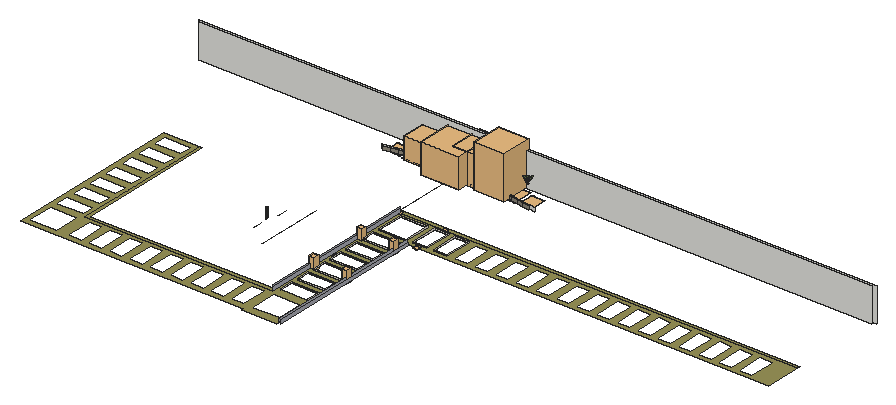
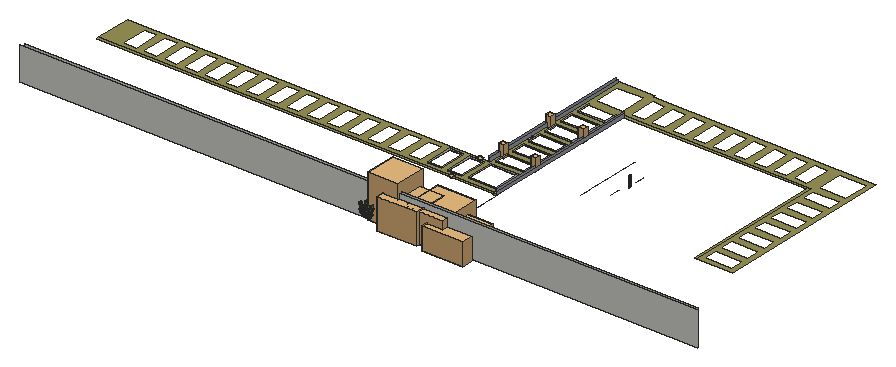
# SketchUp Ruby script. Lengths in inches.
U = 1.inch
M = Sketchup.active_model
def pt(a) = Geom::Point3d.new(a.map { |v| v * U })
def face(e, loops, mat)
  f = e.add_face(loops[0].map { |a| pt(a) })
  loops[1..].each { |l| e.add_face(l.map { |a| pt(a) }).erase! }
  f.material = f.back_material = mat if mat
  f
end
# faces: each face lists its corners as indices into pts; further lists are holes
def faces(e, pts, list, mat = nil) = list.each { |f| face(e, (f[0].is_a?(Array) ? f : [f]).map { |l| l.map { |i| pts[i] } }, mat) }
# xy, xz, yz: faces in a plane at the given z, y or x. An outline is a flat list of corners, or four numbers for a rectangle; further outlines are holes
def ring(l) = l.size == 4 ? [[l[0], l[1]], [l[2], l[1]], [l[2], l[3]], [l[0], l[3]]] : l.each_slice(2).to_a
def flat(e, list, mat, &to3) = list.each { |f| face(e, (f[0].is_a?(Array) ? f : [f]).map { |l| ring(l).map { |u, v| to3.(u, v) } }, mat) }
def xy(e, z, list, mat = nil) = flat(e, list, mat) { |x, y| [x, y, z] }
def xz(e, y, list, mat = nil) = flat(e, list, mat) { |x, z| [x, y, z] }
def yz(e, x, list, mat = nil) = flat(e, list, mat) { |y, z| [x, y, z] }
def lines(e, pts, list) = list.each { |a, b| e.add_line(pt(pts[a]), pt(pts[b])) }
# prism: a flat outline (further loops are holes) pulled along v
def prism(e, loops, v, mat = nil)
  f = face(e, loops, mat); d = Geom::Vector3d.new(v.map { |x| x * U })
  f.pushpull(f.normal.samedirection?(d) ? d.length : -d.length)
end
def box(e, o, s, mat = nil) = prism(e, [[o, [o[0] + s[0], o[1], o[2]], [o[0] + s[0], o[1] + s[1], o[2]], [o[0], o[1] + s[1], o[2]]]], [0, 0, s[2]], mat)
def at(x, y, z, deg = 0) = Geom::Transformation.translation(pt([x, y, z])) * Geom::Transformation.rotation(ORIGIN, Z_AXIS, deg.degrees)
def axes(o, x, y, z) = Geom::Transformation.new([*x, 0, *y, 0, *z, 0, *pt(o).to_a, 1])
def part(name) = M.definitions.add(name)
# library, detail: a bought-in or finely detailed component or shape, given as its bounding box
def library(name, o, s) = part(name).tap { |d| box(d.entities, o, s) }
def detail(e, o, s) = box(e.add_group.entities, o, s)
def put(e, d, t, mat = nil) = e.add_instance(d, t).tap { |i| i.material = mat if mat }
def group(e, t, mat = nil) = e.add_group.tap { |g| g.transformation = t; g.material = mat if mat }.entities
root = M.entities
M.materials.add("Marble_01_1K").color = [230, 221, 211]
M.materials.add("Marble_07_1K").color = [36, 34, 36]
M.materials.add("Marble_20_1K").color = [172, 173, 182]
M.materials.add("Material__4").color = [36, 36, 36]
M.materials.add("Material__6").color = [79, 108, 5]
M.materials.add("Plaster_06_1K").color = [141, 135, 122]
M.materials.add("Soil_04_1K").color = [152, 146, 88]
M.materials.add("calathea lutea").color = [121, 145, 80]
c1 = library("tt",[-12.4,-12.1,0],[24.8,24.2,0.01])
c2 = library("ew",[-14.92,-16.84,0],[29.84,33.68,0.01])
c3 = library("t1",[-17.79,-17.21,0],[35.58,34.42,0.01])
c4 = library("light",[-4,-4,0],[8,8,0.01])
c5 = library("Group\#54",[0,0,0],[2062.46,2062.46,4833.66])
c6 = part("Landscape+Light")
put(c6.entities,c5,at(-2096.57,-1031.23,-3775.98))
c7 = part("Group\#156")
g1 = group(c7.entities,at(8.61,38.85,0))
xy(g1,0,[[0,0,2.82,19.1,22.58,0],[22.58,0,2.82,19.1,22.58,19.1]],"calathea lutea")
p = [[2.82,19.1,0],[7.19,48.22,5.13],[10.77,48.22,5.13],[12.74,48.22,5.13],[22.58,48.22,5.13],[22.58,19.1,0]]
faces(g1,p,[[0,1,2,3,4,5]],"calathea lutea")
g2 = group(c7.entities,at(-0.77,-7.77,0))
p = [[14.8125,23.31,1.46],[21.35,23.31,0],[14.8125,0,1.46],[21.35,0,0],[27.89,0,1.46],[27.89,23.31,1.46],
  [8.27,46.62,2.92],[21.35,46.62,0],[34.4375,46.62,2.92],[4.47,23.31,6.43],[0,0,8.59],[33.76,0,4.28],
  [33.76,23.31,4.28]]
faces(g2,p,[[0,1,2],[3,2,1],[4,3,5],[1,5,3],[6,7,0],[1,0,7],[5,1,8],[7,8,1],
  [9,0,2,10],[11,4,5,12],[9,6,0],[12,5,8]],"calathea lutea")
c8 = part("Group\#150")
xy(c8.entities,0,[[0,0,0,33.87,27.21,33.87,19.71,0]],"calathea lutea")
c9 = part("Group\#157")
xy(c9.entities,1.04,[[21.13,33.87,21.13,57.59,32.375,57.59,27.12,33.87]],"calathea lutea")
xy(c9.entities,1.32,[[0.12,33.87,7.74,57.59]],"calathea lutea")
p = [[7.74,33.87,1.32],[11.8,57.59,0.61],[15.24,57.59,0],[15.24,33.87,0],[18.43,57.59,0.5625],[21.13,57.59,1.04],
  [21.13,33.87,1.04],[15.24,77.7,2.36],[21.13,77.7,3.4],[7.74,57.59,1.32],[7.74,77.7,3.69],[36.83,77.7,3.4],
  [32.375,57.59,1.04],[0.12,57.59,1.32],[0.12,77.7,3.69]]
faces(c9.entities,p,[[0,1,2,3],[3,2,4],[3,4,5,6],[7,2,1],[8,4,2,7],[0,9,1],[7,1,9,10],[8,5,4],
  [11,12,5,8],[10,9,13,14]],"calathea lutea")
put(c9.entities,c8,axes([0,-16.9375,0],[1,0,0],[0,1.5,0],[0,0,1]))
c10 = part("Group\#155")
g3 = group(c10.entities,at(0,-17.3,0))
xy(g3,0,[[0,0,28.07,51.9]],"calathea lutea")
g4 = group(c10.entities,at(0.9,34.6,0))
xy(g4,0,[[13.14,0,13.14,26.22,16.85,26.22],[13.14,0,16.85,26.22,20.16,26.22,20.16,0]],"calathea lutea")
p = [[6.36,0,1.82],[9.95,26.22,0.86],[13.14,26.22,0],[13.14,0,0],[20.16,0,0],[20.16,26.22,0],
  [27.07,26.22,1.22],[27.07,0,1.22],[13.14,49.5625,5.91],[20.16,49.5625,5.91],[16.85,26.22,0],[27.07,49.5625,7.125],
  [6.36,26.22,1.82],[6.36,49.5625,7.72],[0,0,4.78],[0,26.22,4.78],[0,49.5625,10.6875]]
faces(g4,p,[[0,1,2,3],[4,5,6,7],[8,2,1],[9,10,2,8],[9,5,10],[11,6,5,9],[0,12,1],[8,1,12,13],
  [14,15,12,0],[13,12,15,16]],"calathea lutea")
c11 = part("Group\#154")
put(c11.entities,c8,axes([0,-16.9375,0],[1,0,0],[0,1.5,0],[0,0,1]))
g5 = group(c11.entities,at(-0.23,33.4,-0.35))
p = [[15.12,39.14,-19.87],[15.12,20.54,-11.86],[11.68,20.84,-11.33],[21.02,39.66,-18.97],[18.3125,20.82,-11.37],[7.62,21.2,-10.71],
  [7.62,39.8,-18.72],[21.02,21.06,-10.96],[36.72,39.66,-18.97],[32.26,21.06,-10.96],[0,21.2,-10.71],[0,39.8,-18.72],
  [7.62,0.66,1.15],[15.12,0,0],[21.02,0.52,0.9],[27.01,0.52,0.9],[0,0.66,1.15]]
faces(g5,p,[[0,1,2],[3,4,1,0],[0,2,5,6],[3,7,4],[8,9,7,3],[6,5,10,11],[12,2,1,13],[13,1,4],
  [13,4,7,14],[12,5,2],[14,7,9,15],[16,10,5,12]],"calathea lutea")
c12 = part("Foliage cluster")
put(c12.entities,c7,axes([37.24,8.07,75.17],[1,0,0],[0,0.45554,-0.89021],[0,0.89021,0.45554]))
put(c12.entities,c9,axes([69.44,65.48,16.68],[-0.53288,-0.84619,0],[0.14694,-0.09253,0.98481],[-0.83334,0.52478,0.17365]))
put(c12.entities,c10,axes([47.9375,70.43,17.04],[0.74664,-0.66523,0],[0.11552,0.12965,0.98481],[-0.65512,-0.7353,0.17365]))
put(c12.entities,c7,axes([76.19,10.66,75.17],[0.70711,0.70711,0],[-0.32212,0.32212,-0.89021],[-0.62948,0.62948,0.45554]))
put(c12.entities,c7,axes([101.91,40.03,75.17],[0,1,0],[-0.45554,0,-0.89021],[-0.89021,0,0.45554]))
put(c12.entities,c7,axes([99.32,78.99,75.17],[-0.70711,0.70711,0],[-0.32212,-0.32212,-0.89021],[-0.62948,-0.62948,0.45554]))
put(c12.entities,c10,axes([34.81,63.36,17.04],[0.99956,-0.02967,0],[0.00515,0.17357,0.98481],[-0.02922,-0.98437,0.17365]))
put(c12.entities,c10,axes([48,37.4,15.8],[-0.14436,0.98953,0],[-0.40248,-0.05871,0.91355],[0.90398,0.13188,0.40674]))
put(c12.entities,c9,axes([56.87,39.77,12.28],[-0.67695,0.4263,0],[-0.18016,-0.28609,0.72505],[0.38636,0.61353,0.33809]))
put(c12.entities,c9,axes([36.12,43.25,12.28],[0.18947,0.77724,0],[-0.32848,0.08007,0.72505],[0.70442,-0.17172,0.33809]))
put(c12.entities,c11,axes([35.1,54.93,11.375],[0.79719,0.06694,0],[-0.03636,0.43302,0.6717],[0.05621,-0.66934,0.43454]))
put(c12.entities,c9,axes([41.66,47.32,12.28],[0.45082,0.66088,0],[-0.2793,0.19053,0.72505],[0.59896,-0.40858,0.33809]))
put(c12.entities,c9,axes([47.89,59.4,12.28],[0.79719,0.06694,0],[-0.02829,0.33691,0.72505],[0.06067,-0.7225,0.33809]))
put(c12.entities,c11,axes([29.53,49.96,11.375],[0.65692,0.45657,0],[-0.248,0.35682,0.6717],[0.38335,-0.55156,0.43454]))
put(c12.entities,c11,axes([29.9,49.27,12.86],[0.34062,0.72386,0],[-0.22849,0.10752,0.7591],[0.68685,-0.32321,0.25252]))
put(c12.entities,c11,axes([36.33,48.82,8.99],[0.09232,0.62522,0],[-0.3396,0.05015,0.53064],[0.52495,-0.07752,0.34329]))
put(c12.entities,c11,axes([49.82,38.52,8.99],[-0.54622,0.31791,0],[-0.17268,-0.29669,0.53064],[0.26692,0.45862,0.34329]))
put(c12.entities,c11,axes([55.68,39.21,8.99],[-0.632,0.00221,0],[-0.0012,-0.34328,0.53064],[0.00185,0.53064,0.34329]))
c13 = library("Group\#28",[0,0,0],[86.94,78.77,46.4375])
c14 = library("Group\#14",[-978.71,-103.24,719.12],[90.2,76.4,68.29])
c15 = library("Group\#13",[-906.16,-138.28,686.8],[98.25,106.18,75.79])
c16 = library("Group\#202",[-3.47,-2.45,12.47],[53.14,54.93,75.51])
xy(root,0,[[[498.69,562.78,561.69,562.78,561.69,850.66,1202.44,850.66,1202.44,913.66,498.69,913.66,498.69,632.1,166.21,632.1,166.21,885.25,103.21,885.25,103.21,567.28,498.69,567.28],[506.43,856.64,554.43,904.64],[506.43,576.78,554.43,624.64],[111.43,576.78,159.43,624.64],[506.43,820.64,554.43,844.64],[506.43,784.64,554.43,808.64],[506.43,748.64,554.43,772.64],[506.43,712.64,554.43,736.64],[506.43,676.64,554.43,700.64],[506.43,640.64,554.43,664.64],[468.08,576.64,492.08,624.64],[432.08,576.64,456.08,624.64],[396.08,576.64,420.08,624.64],[360.08,576.64,384.08,624.64],[324.08,576.64,348.08,624.64],[288.08,576.64,312.08,624.64],[252.08,576.64,276.08,624.64],[216.08,576.64,240.08,624.64],[180.08,576.64,204.08,624.64],[111.43,636.64,159.43,660.64],[111.43,672.64,159.43,696.64],[111.43,708.64,159.43,732.64],[111.43,744.64,159.43,768.64],[111.43,780.64,159.43,804.64],[111.43,816.64,159.43,840.64],[111.43,852.64,159.43,876.64],[1142.43,858.14,1166.43,906.14],[1106.43,858.14,1130.43,906.14],[1070.43,858.14,1094.43,906.14],[1034.43,858.14,1058.43,906.14],[998.43,858.14,1022.43,906.14],[962.43,858.14,986.43,906.14],[926.43,858.14,950.43,906.14],[890.43,858.14,914.43,906.14],[854.43,858.14,878.43,906.14],[818.43,858.14,842.43,906.14],[782.43,858.14,806.43,906.14],[746.43,858.14,770.43,906.14],[710.43,858.14,734.43,906.14],[674.43,858.14,698.43,906.14],[638.43,858.14,662.43,906.14],[602.43,858.14,626.43,906.14],[566.43,858.14,590.43,906.14]],[166.21,632.1,166.21,885.25,170.71,885.25,170.71,636.6,494.19,636.6,494.19,918.16,1202.44,918.16,1202.44,913.66,498.69,913.66,498.69,632.1]],"Soil_04_1K")
xz(root,664.64,[[506.43,0,554.43,2]],"Marble_01_1K")
xz(root,676.64,[[506.43,0,554.43,2]],"Marble_01_1K")
xz(root,700.64,[[506.43,0,554.43,2]],"Marble_01_1K")
xz(root,712.64,[[506.43,0,554.43,2]],"Marble_01_1K")
xz(root,736.64,[[506.43,0,554.43,2]],"Marble_01_1K")
xz(root,748.64,[[506.43,0,554.43,2]],"Marble_01_1K")
xz(root,772.64,[[506.43,0,554.43,2]],"Marble_01_1K")
xz(root,782.54,[[365.49,0,365.54,18]],"Marble_07_1K")
xz(root,782.55,[[365.375,0,365.4375,18]],"Marble_07_1K")
xz(root,782.65,[[364.85,0,364.91,18]],"Marble_07_1K")
xz(root,784.64,[[506.43,0,554.43,2]],"Marble_01_1K")
xz(root,808.64,[[506.43,0,554.43,2]],"Marble_01_1K")
xz(root,820.64,[[506.43,0,554.43,2]],"Marble_01_1K")
xz(root,844.64,[[506.43,0,554.43,2]],"Marble_01_1K")
xz(root,856.64,[[506.43,0,554.43,2]],"Marble_01_1K")
xz(root,858.14,[[566.43,0,590.43,2],[602.43,0,626.43,2]],"Marble_01_1K")
xz(root,904.64,[[506.43,0,554.43,2]],"Marble_01_1K")
xz(root,906.14,[[566.43,0,590.43,2],[602.43,0,626.43,2]],"Marble_01_1K")
xz(root,1076.74,[[12.46,0,1204.46,60]])
xz(root,1080.74,[[8.46,0,1208.46,60]])
yz(root,364.93,[[783.16,0,783.21,18],[783.21,0,783.26,18]],"Marble_07_1K")
yz(root,364.95,[[786.07,0,786.13,18],[786.13,0,786.18,18]],"Marble_07_1K")
yz(root,365.14,[[786.52,0,786.59,18],[786.59,0,786.63,18]],"Marble_07_1K")
yz(root,365.21,[[784.83,0,784.88,18]],"Marble_07_1K")
yz(root,365.22,[[784.97,0,785.03,18]],"Marble_07_1K")
yz(root,365.23,[[785.09,0,785.14,18],[785.14,0,785.2,18],[785.2,0,785.24,18]],"Marble_07_1K")
yz(root,365.36,[[783.08,0,783.14,18]],"Marble_07_1K")
yz(root,365.65,[[783.76,0,783.81,18]],"Marble_07_1K")
yz(root,494.19,[[636.6,0,918.16,6]],"Marble_20_1K")
yz(root,498.69,[[632.1,0,913.66,6]],"Marble_20_1K")
yz(root,506.43,[[640.64,0,664.64,2],[676.64,0,700.64,2],[712.64,0,736.64,2],[748.64,0,772.64,2],[784.64,0,808.64,2],
  [820.64,0,844.64,2],[856.64,0,904.64,2]],"Marble_01_1K")
yz(root,554.43,[[640.64,0,664.64,2],[676.64,0,700.64,2],[712.64,0,736.64,2],[748.64,0,772.64,2],[784.64,0,808.64,2],
  [820.64,0,844.64,2],[856.64,0,904.64,2]],"Marble_01_1K")
yz(root,561.69,[[567.28,0,850.66,6]],"Marble_20_1K")
yz(root,566.19,[[565.82,0,846.16,6]],"Marble_20_1K")
yz(root,566.43,[[858.14,0,906.14,2]],"Marble_01_1K")
yz(root,590.43,[[858.14,0,906.14,2]],"Marble_01_1K")
yz(root,602.43,[[858.14,0,906.14,2]],"Marble_01_1K")
yz(root,626.43,[[858.14,0,906.14,2]],"Marble_01_1K")
p = [[365.4375,782.55,0],[365.4375,782.55,18],[365.49,782.54,18],[365.49,782.54,0],[365.54,782.54,0],[365.54,782.54,18],
  [365.51,782.62,18],[365.51,782.62,0],[364.91,782.65,0],[364.91,782.65,18],[365.01,782.63,18],[365.01,782.63,0],
  [365.1,782.61,18],[365.1,782.61,0],[365.19,782.6,18],[365.19,782.6,0],[365.29,782.58,18],[365.29,782.58,0],
  [365.375,782.55,18],[365.375,782.55,0],[365.5,782.67,18],[365.5,782.67,0],[364.76,782.74,0],[364.76,782.74,18],
  [364.8,782.7,18],[364.8,782.7,0],[364.85,782.65,18],[364.85,782.65,0],[365.45,782.75,0],[365.45,782.75,18],
  [365.4375,782.78,18],[365.4375,782.78,0],[364.79,782.83,0],[364.79,782.83,18],[364.76,782.79,18],[364.76,782.79,0],
  [364.81,782.88,0],[364.81,782.88,18],[365.42,782.83,0],[365.42,782.83,18],[365.39,782.89,18],[365.39,782.89,0],
  [364.83,782.92,0],[364.83,782.92,18],[364.86,782.97,0],[364.86,782.97,18],[365.375,782.93,0],[365.375,782.93,18],
  [365.36,782.98,18],[365.36,782.98,0],[364.875,783.01,0],[364.875,783.01,18],[364.9,783.07,0],[364.9,783.07,18],
  [365.35,783.03,0],[365.35,783.03,18],[365.36,783.08,18],[365.36,783.08,0],[364.92,783.12,0],[364.92,783.12,18],
  [364.93,783.16,0],[364.93,783.16,18],[365.36,783.14,0],[365.36,783.14,18],[365.38,783.1875,18],[365.38,783.1875,0],
  [365.4,783.24,18],[365.4,783.24,0],[365.42,783.28,18],[365.42,783.28,0],[364.9,783.36,0],[364.9,783.36,18],
  [364.92,783.3,18],[364.92,783.3,0],[364.93,783.26,18],[364.93,783.26,0],[365.44,783.34,18],[365.44,783.34,0],
  [365.47,783.39,18],[365.47,783.39,0],[364.85,783.47,0],[364.85,783.47,18],[364.88,783.42,18],[364.88,783.42,0],
  [365.5,783.45,18],[365.5,783.45,0],[364.81,783.56,0],[364.81,783.56,18],[364.83,783.52,18],[364.83,783.52,0],
  [365.52,783.49,18],[365.52,783.49,0],[365.55,783.55,18],[365.55,783.55,0],[365.58,783.6,18],[365.58,783.6,0],
  [364.77,783.64,0],[364.77,783.64,18],[365.61,783.65,18],[365.61,783.65,0],[365.64,783.7,18],[365.64,783.7,0],
  [365.65,783.76,18],[365.65,783.76,0],[365.65,783.81,0],[365.65,783.81,18],[365.64,783.875,18],[365.64,783.875,0],
  [365.63,783.92,0],[365.63,783.92,18],[365.61,783.98,18],[365.61,783.98,0],[365.59,784.03,0],[365.59,784.03,18],
  [365.56,784.07,18],[365.56,784.07,0],[365.52,784.14,0],[365.52,784.14,18],[365.49,784.18,18],[365.49,784.18,0],
  [365.47,784.22,0],[365.47,784.22,18],[365.43,784.26,18],[365.43,784.26,0],[365.39,784.33,0],[365.39,784.33,18],
  [365.35,784.38,18],[365.35,784.38,0],[365.32,784.41,0],[365.32,784.41,18],[365.28,784.47,18],[365.28,784.47,0],
  [365.26,784.5,0],[365.26,784.5,18],[365.23,784.55,18],[365.23,784.55,0],[365.18,784.64,0],[365.18,784.64,18],
  [365.19,784.69,18],[365.19,784.69,0],[365.21,784.59,0],[365.21,784.59,18],[364.79,784.76,0],[364.79,784.76,18],
  [364.77,784.71,18],[364.77,784.71,0],[365.2,784.74,18],[365.2,784.74,0],[365.19,784.79,18],[365.19,784.79,0],
  [364.82,784.8125,0],[364.82,784.8125,18],[364.84,784.86,0],[364.84,784.86,18],[365.21,784.83,18],[365.21,784.83,0],
  [364.85,784.9,0],[364.85,784.9,18],[364.87,784.95,0],[364.87,784.95,18],[365.21,784.88,0],[365.21,784.88,18],
  [365.2,784.92,18],[365.2,784.92,0],[365.22,784.97,18],[365.22,784.97,0],[364.86,785.05,0],[364.86,785.05,18],
  [364.88,785.01,18],[364.88,785.01,0],[365.22,785.03,0],[365.22,785.03,18],[365.23,785.09,18],[365.23,785.09,0],
  [364.8,785.16,0],[364.8,785.16,18],[364.83,785.11,18],[364.83,785.11,0],[364.78,785.2,0],[364.78,785.2,18],
  [365.23,785.24,0],[365.23,785.24,18],[365.22,785.29,18],[365.22,785.29,0],[365.2,785.35,18],[365.2,785.35,0],
  [365.18,785.4375,0],[365.18,785.4375,18],[365.17,785.49,18],[365.17,785.49,0],[365.19,785.39,0],[365.19,785.39,18],
  [365.15,785.54,0],[365.15,785.54,18],[365.14,785.59,18],[365.14,785.59,0],[365.13,785.64,0],[365.13,785.64,18],
  [365.11,785.7,18],[365.11,785.7,0],[365.1,785.74,0],[365.1,785.74,18],[365.09,785.78,18],[365.09,785.78,0],
  [365.07,785.84,0],[365.07,785.84,18],[365.04,785.89,18],[365.04,785.89,0],[365.02,785.93,0],[365.02,785.93,18],
  [364.99,785.97,18],[364.99,785.97,0],[364.96,786.02,0],[364.96,786.02,18],[364.95,786.07,18],[364.95,786.07,0],
  [364.95,786.18,0],[364.95,786.18,18],[364.97,786.23,18],[364.97,786.23,0],[364.99,786.28,18],[364.99,786.28,0],
  [365.02,786.33,18],[365.02,786.33,0],[365.03,786.37,18],[365.03,786.37,0],[365.06,786.41,18],[365.06,786.41,0],
  [365.09,786.44,18],[365.09,786.44,0],[365.12,786.48,18],[365.12,786.48,0],[365.14,786.52,18],[365.14,786.52,0],
  [365.14,786.63,0],[365.14,786.63,18],[365.13,786.6875,18],[365.13,786.6875,0],[365.1,786.74,0],[365.1,786.74,18],
  [365.08,786.78,18],[365.08,786.78,0],[365.05,786.83,0],[365.05,786.83,18],[365.01,786.87,18],[365.01,786.87,0],
  [364.97,786.92,0],[364.97,786.92,18],[364.9375,786.95,18],[364.9375,786.95,0],[364.86,787.05,0],[364.86,787.05,18],
  [364.83,787.07,18],[364.83,787.07,0],[364.9,786.99,0],[364.9,786.99,18],[364.79,787.11,0],[364.79,787.11,18],
  [364.75,787.17,18],[364.75,787.17,0],[621.54,1031.93,0],[632.59,1030.19,0],[632.59,1030.19,6],[621.54,1031.93,6],
  [643.01,1031.82,0],[632.4,1033.25,0],[632.4,1033.25,6],[643.01,1031.82,6],[610.49,1033.89,0],[610.49,1033.89,6],
  [621.78,1034.93,0],[621.78,1034.93,6],[599.44,1036.01,0],[599.44,1036.01,6],[611.16,1036.82,0],[611.16,1036.82,6],
  [588.39,1038.24,0],[588.39,1038.24,6],[600.52,1038.86,0],[600.52,1038.86,6],[368.91,1037.36,0],[381.01,1039.59,0],
  [381.01,1039.59,6],[368.91,1037.36,6],[577.32,1040.51,0],[577.32,1040.51,6],[589.85,1041,0],[589.85,1041,6],
  [393.07,1041.98,0],[393.07,1041.98,6],[377.04,1041.89,0],[365.4,1039.79,0],[365.4,1039.79,6],[377.04,1041.89,6],
  [566.22,1042.77,0],[566.22,1042.77,6],[579.16,1043.19,0],[579.16,1043.19,6],[388.68,1044.16,0],[388.68,1044.16,6],
  [405.09,1044.41,0],[405.09,1044.41,6],[555.1,1044.96,0],[555.1,1044.96,6],[568.4375,1045.38,0],[568.4375,1045.38,6],
  [400.3,1046.5,0],[400.3,1046.5,6],[417.0625,1046.76,0],[417.0625,1046.76,6],[543.94,1047.03,0],[543.94,1047.03,6],
  [557.67,1047.52,0],[557.67,1047.52,6],[411.91,1048.82,0],[411.91,1048.82,6],[428.97,1048.93,0],[428.97,1048.93,6],
  [532.74,1048.91,0],[532.74,1048.91,6],[546.86,1049.55,0],[546.86,1049.55,6],[423.48,1051.01,0],[423.48,1051.01,6],
  [440.82,1050.8125,0],[440.82,1050.8125,6],[521.49,1050.5625,0],[521.49,1050.5625,6],[536,1051.43,0],[536,1051.43,6],
  [510.1875,1051.92,0],[510.1875,1051.92,6],[452.59,1052.29,0],[452.59,1052.29,6],[435.03,1052.97,0],[435.03,1052.97,6],
  [525.07,1053.1,0],[525.07,1053.1,6],[498.82,1052.92,0],[498.82,1052.92,6],[464.27,1053.25,0],[464.27,1053.25,6],
  [487.38,1053.51,0],[487.38,1053.51,6],[446.53,1054.61,0],[446.53,1054.61,6],[514.09,1054.51,0],[514.09,1054.51,6],
  [475.87,1053.64,0],[475.87,1053.64,6],[503.03,1055.6,0],[503.03,1055.6,6],[457.99,1055.8125,0],[457.99,1055.8125,6],
  [491.9,1056.34,0],[491.9,1056.34,6],[469.38,1056.49,0],[469.38,1056.49,6],[480.68,1056.65,0],[480.68,1056.65,6],
  [494.19,918.16,0],[494.19,1053.16,0],[404.37,845.62,0],[404.37,725.46,0],[372.1,819.24,0],[372.1,817.02,0],
  [372.12,817.02,0],[366.875,752.88,0],[366.875,755.1,0],[366.89,755.1,0],[372.1,800.9375,0],[366.875,771.18,0]]
faces(root,p,[[0,1,2,3],[4,5,6,7],[8,9,10,11],[11,10,12,13],[13,12,14,15],[15,14,16,17],[17,16,18,19],[7,6,20,21],
  [22,23,24,25],[25,24,26,27],[28,29,30,31],[21,20,29,28],[32,33,34,35],[36,37,33,32],[38,39,40,41],[31,30,39,38],
  [42,43,37,36],[44,45,43,42],[46,47,48,49],[41,40,47,46],[50,51,45,44],[52,53,51,50],[54,55,56,57],[49,48,55,54],
  [58,59,53,52],[60,61,59,58],[62,63,64,65],[65,64,66,67],[67,66,68,69],[70,71,72,73],[73,72,74,75],[69,68,76,77],
  [77,76,78,79],[80,81,82,83],[83,82,71,70],[79,78,84,85],[86,87,88,89],[89,88,81,80],[85,84,90,91],[91,90,92,93],
  [93,92,94,95],[96,97,87,86],[95,94,98,99],[99,98,100,101],[101,100,102,103],[104,105,106,107],[108,109,110,111],[107,106,109,108],
  [112,113,114,115],[111,110,113,112],[116,117,118,119],[115,114,117,116],[120,121,122,123],[119,118,121,120],[124,125,126,127],[123,122,125,124],
  [128,129,130,131],[127,126,129,128],[132,133,134,135],[131,130,133,132],[136,137,138,139],[140,141,137,136],[135,134,141,140],[142,143,144,145],
  [139,138,146,147],[147,146,148,149],[150,151,143,142],[152,153,151,150],[149,148,154,155],[156,157,153,152],[158,159,157,156],[160,161,162,163],
  [163,162,164,165],[166,167,168,169],[169,168,159,158],[170,171,172,173],[174,175,176,177],[177,176,167,166],[178,179,175,174],[180,181,182,183],
  [183,182,184,185],[186,187,188,189],[190,191,187,186],[185,184,191,190],[192,193,194,195],[189,188,193,192],[196,197,198,199],[195,194,197,196],
  [200,201,202,203],[199,198,201,200],[204,205,206,207],[203,202,205,204],[208,209,210,211],[207,206,209,208],[212,213,214,215],[211,210,213,212],
  [216,217,218,219],[219,218,220,221],[221,220,222,223],[223,222,224,225],[225,224,226,227],[227,226,228,229],[229,228,230,231],[231,230,232,233],
  [234,235,236,237],[238,239,240,241],[237,236,239,238],[242,243,244,245],[241,240,243,242],[246,247,248,249],[245,244,247,246],[250,251,252,253],
  [254,255,251,250],[249,248,255,254],[256,257,258,259],[253,252,257,256]],"Marble_07_1K")
faces(root,p,[[260,261,262,263],[268,260,263,269],[272,268,269,273],[276,272,273,277],[280,281,282,283],[284,276,277,285],[281,288,289,282],[294,284,285,295],
  [288,300,301,289],[302,294,295,303],[300,308,309,301],[310,302,303,311],[308,316,317,309],[318,310,311,319],[316,324,325,317],[326,318,319,327],
  [330,326,327,331],[324,332,333,325],[338,330,331,339],[332,340,341,333],[342,338,339,343],[340,348,349,341],[348,342,343,349]],"Plaster_06_1K")
faces(root,p,[[264,265,266,267],[265,270,271,266],[270,274,275,271],[274,278,279,275],[278,286,287,279],[290,291,292,293],[286,296,297,287],[298,290,293,299],
  [296,304,305,297],[306,298,299,307],[304,312,313,305],[314,306,307,315],[312,320,321,313],[322,314,315,323],[320,328,329,321],[334,322,323,335],
  [328,336,337,329],[344,334,335,345],[336,346,347,337],[346,350,351,347],[352,344,345,353],[350,354,355,351],[356,352,353,357],[354,358,359,355],
  [358,356,357,359]])
lines(root,p,[[360,361],[362,363],[364,365],[365,366],[367,368],[368,369],[365,370],[368,371]])
put(root,c1,at(385.58,1051.8125,0,90))
put(root,c2,at(422.02,1050.15,0,90))
put(root,c3,at(466.26,1052.3,0,90))
put(root,c4,at(498.19,763.07,0,90))
put(root,c4,at(498.375,913.8,0))
put(root,c6,axes([501.78,714.02,13.79],[0,-0.0044,0],[0.0044,0,0],[0,0,0.0044]))
put(root,c6,axes([501.78,818.49,13.79],[0,-0.0044,0],[0.0044,0,0],[0,0,0.0044]))
put(root,c1,at(507.92,1051.8125,0,90))
g6 = group(root,at(407.99,1017.59,-3))
put(g6,c12,axes([161.54,64.35,6.01],[0.19523,-0.19694,0],[0.19694,0.19523,0],[0,0,0.24957]))
put(g6,c13,axes([0,18.48,0.92],[0.83,0,0],[0,0.83,0],[0,0,0.83]))
put(g6,c14,axes([859.63,98.87,-568.1],[0.79,0,0],[0,0.79,0],[0,0,0.79]),"Material__4")
put(g6,c15,axes([669.69,95.42,-472.48],[0.69,0,0],[0,0.69,0],[0,0,0.69]),"Material__6")
put(g6,c16,at(133.52,12.51,-9.6))
put(root,c2,at(544.36,1050.15,0,90))
put(root,c6,axes([559.29,714.02,13.79],[0,-0.0044,0],[0.0044,0,0],[0,0,0.0044]))
put(root,c6,axes([559.29,818.49,13.79],[0,-0.0044,0],[0.0044,0,0],[0,0,0.0044]))
put(root,c4,at(561.9,763.07,0,90))
put(root,c4,at(578.43,850.3,0))
put(root,c4,at(578.43,913.8,0))
put(root,c3,at(588.6,1052.3,0,90))
put(root,c1,at(623.12,1051.8125,0,90))
